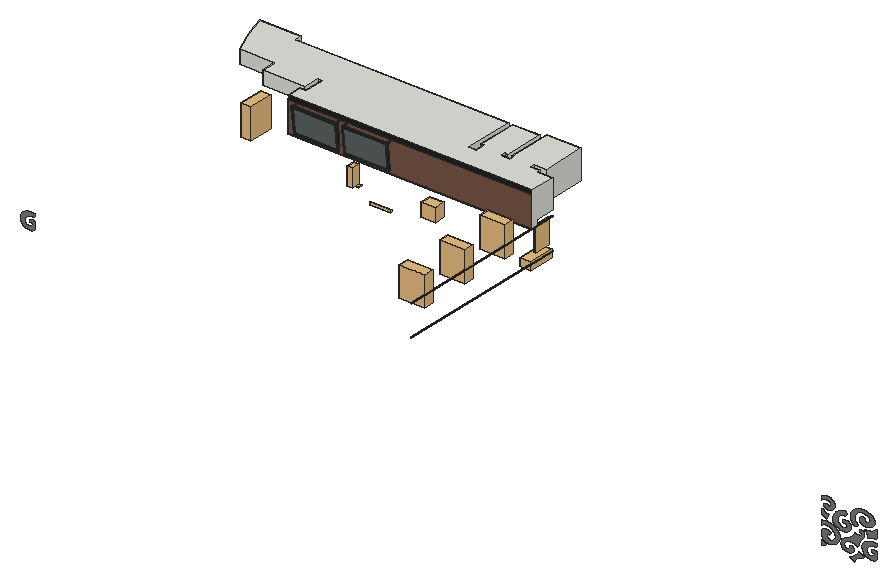
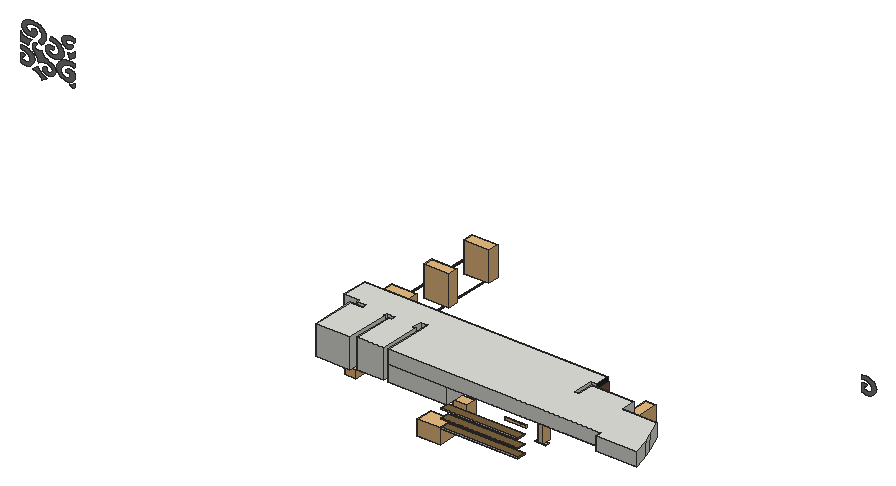
# SketchUp Ruby script. Lengths in inches.
U = 1.inch
M = Sketchup.active_model
def pt(a) = Geom::Point3d.new(a.map { |v| v * U })
def face(e, loops, mat)
  f = e.add_face(loops[0].map { |a| pt(a) })
  loops[1..].each { |l| e.add_face(l.map { |a| pt(a) }).erase! }
  f.material = f.back_material = mat if mat
  f
end
# faces: each face lists its corners as indices into pts; further lists are holes
def faces(e, pts, list, mat = nil) = list.each { |f| face(e, (f[0].is_a?(Array) ? f : [f]).map { |l| l.map { |i| pts[i] } }, mat) }
# xy, xz, yz: faces in a plane at the given z, y or x. An outline is a flat list of corners, or four numbers for a rectangle; further outlines are holes
def ring(l) = l.size == 4 ? [[l[0], l[1]], [l[2], l[1]], [l[2], l[3]], [l[0], l[3]]] : l.each_slice(2).to_a
def flat(e, list, mat, &to3) = list.each { |f| face(e, (f[0].is_a?(Array) ? f : [f]).map { |l| ring(l).map { |u, v| to3.(u, v) } }, mat) }
def xy(e, z, list, mat = nil) = flat(e, list, mat) { |x, y| [x, y, z] }
def xz(e, y, list, mat = nil) = flat(e, list, mat) { |x, z| [x, y, z] }
def yz(e, x, list, mat = nil) = flat(e, list, mat) { |y, z| [x, y, z] }
def lines(e, pts, list) = list.each { |a, b| e.add_line(pt(pts[a]), pt(pts[b])) }
# prism: a flat outline (further loops are holes) pulled along v
def prism(e, loops, v, mat = nil)
  f = face(e, loops, mat); d = Geom::Vector3d.new(v.map { |x| x * U })
  f.pushpull(f.normal.samedirection?(d) ? d.length : -d.length)
end
def box(e, o, s, mat = nil) = prism(e, [[o, [o[0] + s[0], o[1], o[2]], [o[0] + s[0], o[1] + s[1], o[2]], [o[0], o[1] + s[1], o[2]]]], [0, 0, s[2]], mat)
def at(x, y, z, deg = 0) = Geom::Transformation.translation(pt([x, y, z])) * Geom::Transformation.rotation(ORIGIN, Z_AXIS, deg.degrees)
def axes(o, x, y, z) = Geom::Transformation.new([*x, 0, *y, 0, *z, 0, *pt(o).to_a, 1])
def part(name) = M.definitions.add(name)
# library, detail: a bought-in or finely detailed component or shape, given as its bounding box
def library(name, o, s) = part(name).tap { |d| box(d.entities, o, s) }
def detail(e, o, s) = box(e.add_group.entities, o, s)
def put(e, d, t, mat = nil) = e.add_instance(d, t).tap { |i| i.material = mat if mat }
def group(e, t, mat = nil) = e.add_group.tap { |g| g.transformation = t; g.material = mat if mat }.entities
root = M.entities
M.materials.add("Floor board").color = [119, 86, 70]
M.materials.add("Floor board2").color = [119, 86, 70]
M.materials.add("Image2").color = [96, 104, 104]
M.materials.add("Material31 copy1").color = [126, 98, 61]
M.materials.add("Small-Wooden-Floor").color = [116, 79, 55]
M.materials.add("Sophie_Shoes2").color = [35, 35, 35]
M.materials.add("[0043_SaddleBrown]4").color = [124, 123, 122]
M.materials.add("[Metal_Corrogated_Shiny]2").color = [193, 193, 193]
c1 = library("Group\#90",[0,0,0],[37.3,15.24,44.88])
c2 = part("Group\#62")
box(c2.entities,[0,-3.9375,0],[1.97,3.9375,1.97],"Sophie_Shoes2")
c3 = part("Component\#73")
detail(c3.entities,[0,0,-0.5],[5.95,16.95,0.625])
c4 = part("omponent_2\#3")
xy(c4.entities,0.125,[[[0.47,0.47,5.47,16.47],[1.375,15.02,4.5625,15.45],[1.375,14.15,4.5625,14.59],[1.375,13.29,4.5625,13.72],[1.375,12.43,4.5625,12.86],[1.375,11.5625,4.5625,12],[1.375,10.7,4.5625,11.13],[1.375,9.84,4.5625,10.27],[1.375,8.97,4.5625,9.41],[1.375,8.11,4.5625,8.54],[1.375,7.25,4.5625,7.68],[1.375,6.38,4.5625,6.82],[1.375,5.52,4.5625,5.95],[1.375,4.66,4.5625,5.09],[1.375,3.79,4.5625,4.23],[1.375,2.93,4.5625,3.36],[1.375,2.07,4.5625,2.5],[1.375,1.26,4.5625,1.64]]],"[Metal_Corrogated_Shiny]2")
put(c4.entities,c3,at(0,0,0))
c5 = library("Cobra Beer Dispense Font",[-3.83,-2.55,-1.15],[8.17,12.19,26.9])
c6 = part("Group\#60")
xy(c6.entities,0,[[-106.3,12.99,7.875,25.59]])
xy(c6.entities,1.97,[[-106.3,12.99,7.875,25.59]],"Material31 copy1")
xz(c6.entities,12.99,[[-106.3,0,7.875,1.97]],"Material31 copy1")
xz(c6.entities,25.59,[[-106.3,0,7.875,1.97]])
yz(c6.entities,-106.3,[[12.99,0,25.59,1.97]],"Material31 copy1")
yz(c6.entities,7.875,[[12.99,0,25.59,1.97]],"Material31 copy1")
c7 = library("IKEA FINTORP-",[6.23,0.25,8.28],[1.42,31.37,3.33])
c8 = library("maq caf expresso 2 mdulos",[-0.08,-0.31,0.08],[34.26,25.22,21.95])
c9 = library("ZJ8P4AC",[-1.97,-16.1,36],[20.97,16.1,19.66])
c10 = library("Group\#93",[0,0,0],[37.3,15.24,44.88])
c11 = library("Group\#94",[0,0,0],[37.3,15.24,44.88])
c12 = library("Group\#105",[0,0,0],[37.34,15.24,44.88])
c13 = library("Group\#84",[0,-1.97,0],[16.33,39.37,11.37])
c14 = library("Group\#83",[-2.91,0,0],[33.89,3.125,48.37])
xz(root,589.17,[[4168.05,173.83,4167.56,174.24,4167.0625,174.64,4166.54,175.02,4166,175.39,4165.4375,175.74,4164.86,176.08,4164.26,176.4,4163.65,176.71,4163.02,177,4162.38,177.27,4161.73,177.53,4161.0625,177.77,4162.625,178.34,4164.13,178.99,4165.5625,179.72,4166.92,180.52,4168.2,181.39,4169.39,182.32,4170.48,183.31,4171.47,184.35,4172.36,185.44,4173.14,186.58,4173.8,187.75,4174.35,188.95,4174.9,188.49,4175.46,188.03,4176.03,187.59,4176.61,187.15,4177.2,186.72,4177.8,186.29,4178.42,185.87,4179.04,185.46,4179.66,185.06,4180.3,184.66,4180.95,184.27,4181.61,183.89,4179.94,183.57,4178.33,183.14,4176.79,182.59,4175.33,181.94,4173.96,181.19,4172.71,180.35,4171.57,179.42,4170.57,178.41,4169.71,177.34,4168.99,176.21,4168.44,175.04],[4119.85,179.89,4119.85,185.26,4120.27,184.92,4120.7,184.6,4121.16,184.3,4121.63,184.01,4122.125,183.73,4122.63,183.47,4123.15,183.23,4123.69,183,4124.24,182.79,4124.81,182.6,4125.38,182.42,4125.97,182.27,4125.59,181.9375,4125.17,181.63,4124.73,181.34,4124.27,181.07,4123.77,180.83,4123.26,180.61,4122.72,180.42,4122.17,180.26,4121.61,180.12,4121.03,180.02,4120.44,179.9375],[4157.27,183.24,4155.84,183.36,4154.45,183.65,4153.14,184.08,4151.93,184.65,4150.86,185.34,4149.94,186.15,4149.21,187.04,4148.67,188.01,4148.34,189.02,4148.23,190.0625,4148.12,191.26,4148.18,192.46,4148.42,193.65,4148.82,194.8125,4149.39,195.9375,4150.11,197.02,4150.99,198.04,4152.01,198.99,4153.16,199.85,4154.43,200.63,4155.81,201.31,4157.27,201.88,4158.66,202.4,4159.99,202.99,4161.27,203.65,4162.47,204.37,4163.6,205.15,4164.65,205.98,4165.62,206.87,4166.5,207.81,4167.28,208.78,4167.96,209.8,4168.55,210.85,4169.02,211.92,4169.7,211.55,4170.44,211.25,4171.23,211.03,4172.06,210.88,4172.9,210.82,4173.75,210.84,4174.59,210.9375,4175.4,211.12,4176.17,211.38,4176.88,211.72,4177.53,212.12,4178.09,212.58,4178.3,212.95,4178.44,213.33,4178.53,213.73,4178.55,214.13,4178.51,214.53,4178.41,214.92,4178.25,215.3,4178.03,215.67,4177.75,216.02,4177.42,216.34,4177.04,216.63,4176.62,216.89,4176.39,217.04,4176.21,217.23,4176.08,217.43,4176,217.65,4175.99,217.875,4176.04,218.1,4176.15,218.3125,4176.32,218.5,4176.53,218.67,4176.78,218.8,4177.07,218.9,4177.37,218.95,4177.93,218.98,4178.48,218.95,4179.03,218.86,4179.55,218.72,4180.04,218.52,4180.48,218.28,4180.875,217.99,4181.21,217.67,4181.47,217.3125,4181.66,216.9375,4181.78,216.54,4181.82,216.14,4182.03,215.47,4182.18,214.79,4182.25,214.11,4182.26,213.42,4182.2,212.73,4182.07,212.05,4181.87,211.38,4181.6,210.72,4181.27,210.08,4180.87,209.45,4180.41,208.85,4179.89,208.27,4178.96,207.26,4178.09,206.23,4177.28,205.16,4176.54,204.07,4175.88,202.95,4175.28,201.82,4174.76,200.67,4174.3,199.5,4173.93,198.32,4173.625,197.12,4173.4,195.92,4173.25,194.71,4172.28,195.61,4171.16,196.41,4169.9,197.09,4168.54,197.66,4167.08,198.09,4165.56,198.375,4163.99,198.52,4162.42,198.52,4160.86,198.37,4159.34,198.07,4157.88,197.63,4156.52,197.0625,4155.54,196.53,4154.68,195.9,4153.93,195.2,4153.31,194.44,4152.83,193.625,4152.5,192.77,4152.32,191.9,4152.31,191.01,4152.45,190.14,4152.75,189.28,4153.19,188.46,4153.78,187.68,4154.33,187.38,4154.93,187.15,4155.57,186.98,4156.24,186.89,4156.93,186.87,4157.61,186.92,4158.27,187.04,4158.89,187.24,4159.48,187.5,4160,187.82,4160.44,188.1875,4160.8125,188.6,4160.69,188.9,4160.6,189.2,4160.55,189.5,4160.53,189.81,4160.55,190.12,4160.59,190.42,4160.67,190.72,4160.79,191.02,4160.94,191.31,4161.11,191.59,4161.32,191.86,4161.56,192.11,4161.79,192.31,4162.0625,192.48,4162.37,192.61,4162.7,192.71,4163.05,192.77,4163.4,192.79,4163.76,192.77,4164.11,192.71,4164.44,192.61,4164.75,192.48,4165.02,192.31,4165.25,192.11,4165.92,191.31,4166.4,190.43,4166.65,189.51,4166.6875,188.57,4166.5,187.63,4166.09,186.74,4165.48,185.91,4164.68,185.17,4163.71,184.53,4162.61,184.03,4161.41,183.66,4160.14,183.45,4158.72,183.27],[4130,184.38,4128.84,184.54,4127.71,184.78,4126.61,185.09,4125.5625,185.48,4124.57,185.94,4123.64,186.47,4122.78,187.05,4122.01,187.69,4121.32,188.38,4120.73,189.12,4120.24,189.89,4119.85,190.7,4119.85,198.78,4120.38,199.6875,4121.16,200.5,4122.14,201.17,4123.3,201.69,4124.58,202.03,4125.93,202.17,4127.29,202.12,4128.61,201.86,4129.82,201.42,4130.89,200.8,4131.76,200.05,4132.4,199.18,4132.49,198.97,4132.54,198.75,4132.55,198.53,4132.51,198.32,4132.42,198.1,4132.3,197.9,4132.13,197.72,4131.93,197.55,4131.7,197.41,4131.44,197.3,4131.16,197.21,4130.87,197.15,4130.14,197.24,4129.4,197.23,4128.68,197.13,4128,196.93,4127.38,196.64,4126.84,196.28,4126.41,195.85,4126.09,195.37,4125.9,194.85,4125.85,194.32,4125.93,193.8,4126.15,193.29,4126.33,192.63,4126.65,192,4127.11,191.41,4127.69,190.88,4128.38,190.43,4129.16,190.06,4130.01,189.78,4130.91,189.6,4131.84,189.53,4132.77,189.5625,4133.68,189.7,4134.55,189.9375,4135.91,190.72,4137.1,191.64,4138.09,192.67,4138.88,193.79,4139.4375,194.98,4139.75,196.21,4139.83,197.47,4139.65,198.72,4139.24,199.93,4138.58,201.1,4137.71,202.18,4136.63,203.17,4136.19,203.82,4135.68,204.45,4135.1,205.04,4134.45,205.59,4133.74,206.1,4132.97,206.57,4132.15,206.99,4131.29,207.37,4130.39,207.68,4129.45,207.94,4128.48,208.15,4127.5,208.3,4126.8,208.36,4126.09,208.375,4125.39,208.35,4124.6875,208.28,4124,208.17,4123.32,208.02,4122.67,207.83,4122.04,207.6,4121.4375,207.33,4120.87,207.03,4120.34,206.69,4119.85,206.32,4119.85,211.9,4122,212.41,4124.21,212.74,4126.47,212.875,4128.73,212.8125,4130.96,212.56,4133.14,212.11,4135.22,211.48,4137.1875,210.67,4139.01,209.7,4140.65,208.58,4142.1,207.33,4143.32,205.96,4144.99,203.92,4146.15,201.7,4146.76,199.375,4146.81,197.01,4146.28,194.67,4145.21,192.43,4143.62,190.36,4141.5625,188.51,4139.09,186.95,4136.28,185.72,4133.22,184.86],[2942.18,185,2940.82,185.0625,2939.48,185.24,2938.1875,185.54,2936.95,185.94,2935.8,186.46,2934.74,187.07,2933.84,187.69,2933.01,188.36,2932.24,189.0625,2931.53,189.8,2930.9,190.57,2930.34,191.375,2929.86,192.2,2929.45,193.05,2929.125,193.92,2928.88,194.79,2928.72,195.68,2928.64,196.58,2928.75,198.46,2929.26,200.32,2930.15,202.09,2931.4,203.75,2932.98,205.26,2934.86,206.58,2936.99,207.67,2939.33,208.53,2941.82,209.12,2944.4,209.4375,2947.02,209.47,2949.62,209.22,2949.62,204.51,2947.39,204.57,2945.18,204.34,2943.06,203.84,2941.09,203.08,2939.33,202.09,2937.84,200.89,2936.66,199.53,2935.83,198.03,2935.37,196.46,2935.3,194.85,2935.62,193.26,2936.3125,191.73,2937.11,191.08,2938.06,190.54,2939.13,190.15,2940.29,189.91,2941.49,189.83,2942.7,189.91,2943.85,190.16,2944.93,190.55,2945.875,191.09,2946.67,191.75,2947.28,192.5,2947.68,193.32,2947.75,193.65,2947.74,193.99,2947.66,194.32,2947.49,194.64,2947.25,194.93,2946.95,195.19,2946.59,195.4,2946.1875,195.57,2945.75,195.6875,2945.29,195.75,2944.82,195.75,2944.36,195.7,2944.12,195.77,2943.89,195.87,2943.68,195.98,2943.48,196.11,2943.31,196.25,2943.15,196.41,2943.03,196.58,2942.92,196.75,2942.85,196.93,2942.8,197.12,2942.78,197.3125,2942.79,197.5,2943.15,197.89,2943.59,198.24,2944.09,198.54,2944.64,198.8,2945.23,199,2945.85,199.14,2946.49,199.22,2947.14,199.24,2947.79,199.19,2948.43,199.09,2949.04,198.93,2949.62,198.7,2949.62,187.07,2948.55,186.46,2947.4,185.94,2946.16,185.54,2944.87,185.24,2943.53,185.0625],
  [4192.8,185,4191.44,185.0625,4190.11,185.24,4188.8125,185.54,4187.58,185.94,4186.42,186.46,4185.36,187.07,4184.47,187.69,4183.63,188.36,4182.86,189.0625,4182.16,189.8,4181.53,190.57,4180.97,191.375,4180.48,192.2,4180.08,193.05,4179.75,193.92,4179.51,194.79,4179.34,195.68,4179.26,196.58,4179.38,198.46,4179.89,200.32,4180.78,202.09,4182.03,203.75,4183.61,205.26,4185.49,206.58,4187.62,207.67,4189.95,208.53,4192.44,209.12,4195.03,209.4375,4197.64,209.47,4200.24,209.22,4200.24,204.51,4198.01,204.57,4195.8,204.34,4193.68,203.84,4191.71,203.08,4189.96,202.09,4188.47,200.89,4187.29,199.53,4186.46,198.03,4186,196.46,4185.92,194.85,4186.24,193.26,4186.9375,191.73,4187.73,191.08,4188.68,190.54,4189.76,190.15,4190.92,189.91,4192.12,189.83,4193.32,189.91,4194.48,190.16,4195.55,190.55,4196.5,191.09,4197.29,191.75,4197.9,192.5,4198.3,193.32,4198.375,193.65,4198.37,193.99,4198.28,194.32,4198.12,194.64,4197.88,194.93,4197.58,195.19,4197.22,195.4,4196.8125,195.57,4196.375,195.6875,4195.91,195.75,4195.45,195.75,4194.98,195.7,4194.74,195.77,4194.51,195.87,4194.3,195.98,4194.11,196.11,4193.93,196.25,4193.78,196.41,4193.65,196.58,4193.55,196.75,4193.47,196.93,4193.42,197.12,4193.4,197.3125,4193.41,197.5,4193.78,197.89,4194.22,198.24,4194.71,198.54,4195.26,198.8,4195.85,199,4196.48,199.14,4197.12,199.22,4197.77,199.24,4198.42,199.19,4199.05,199.09,4199.67,198.93,4200.24,198.7,4200.24,187.07,4199.18,186.46,4198.02,185.94,4196.79,185.54,4195.49,185.24,4194.16,185.0625],[4150.69,208.61,4148.36,208.71,4146.07,209.07,4143.89,209.68,4141.87,210.53,4140.0625,211.6,4138.5,212.86,4137.24,214.28,4136.29,215.82,4135.69,217.45,4135.45,219.125,4135.58,220.81,4136.07,222.46,4136.625,224.06,4137.38,225.62,4138.33,227.12,4139.47,228.55,4140.79,229.9,4142.27,231.16,4143.91,232.31,4145.69,233.35,4147.59,234.27,4149.6,235.06,4151.7,235.71,4153.875,236.22,4154.29,235.77,4154.65,235.31,4154.96,234.82,4155.23,234.32,4155.4375,233.81,4155.59,233.28,4155.69,232.75,4155.74,232.22,4155.73,231.68,4155.66,231.15,4155.54,230.62,4155.37,230.1,4154.01,230.21,4152.65,230.19,4151.31,230.04,4150.01,229.75,4148.78,229.33,4147.63,228.8,4146.61,228.16,4145.71,227.42,4144.96,226.6,4144.38,225.71,4143.97,224.77,4143.75,223.8,4143.38,222.89,4143.15,221.95,4143.0625,221,4143.12,220.05,4143.31,219.11,4143.64,218.19,4144.11,217.3,4144.7,216.45,4145.42,215.65,4146.26,214.91,4147.19,214.24,4148.23,213.65,4149.18,213.25,4150.23,212.99,4151.32,212.875,4152.43,212.91,4153.5,213.1,4154.51,213.43,4155.41,213.89,4156.18,214.46,4156.78,215.13,4157.19,215.875,4157.41,216.66,4157.41,217.45,4157.32,217.85,4157.16,218.23,4156.93,218.59,4156.63,218.92,4156.28,219.23,4155.86,219.49,4155.41,219.71,4154.91,219.89,4154.39,220.01,4153.85,220.09,4153.29,220.1,4152.74,220.07,4152.17,220.05,4151.61,220.13,4151.08,220.3,4150.62,220.55,4150.25,220.86,4150,221.23,4149.86,221.63,4149.86,222.05,4149.98,222.45,4150.23,222.83,4150.59,223.15,4151.04,223.4,4152.29,223.84,4153.63,224.12,4155.01,224.21,4156.39,224.12,4157.73,223.85,4158.98,223.4,4160.09,222.81,4161.04,222.07,4161.78,221.23,4162.31,220.3,4162.58,219.32,4162.61,218.32,4162.66,217.11,4162.49,215.9,4162.08,214.72,4161.46,213.6,4160.625,212.54,4159.6,211.58,4158.4,210.73,4157.05,210.01,4155.58,209.42,4154.01,208.99,4152.37,208.72],[4188.26,213.07,4188.16,213.85,4188,214.62,4187.78,215.39,4187.52,216.14,4187.2,216.89,4186.82,217.625,4186.4,218.34,4185.93,219.05,4185.4,219.73,4184.83,220.4,4184.22,221.04,4183.56,221.66,4185.21,221.55,4186.87,221.5625,4188.52,221.7,4190.14,221.96,4191.72,222.33,4193.24,222.82,4194.68,223.41,4196.03,224.11,4197.27,224.91,4198.39,225.79,4199.39,226.75,4200.24,227.78,4200.24,215.23,4199.2,215.21,4198.17,215.16,4197.13,215.08,4196.1,214.98,4195.08,214.84,4194.07,214.67,4193.07,214.47,4192.08,214.25,4191.1,213.99,4190.14,213.71,4189.1875,213.41],[4127.19,216.375,4126.5,216.63,4125.81,216.91,4125.14,217.2,4124.48,217.52,4123.84,217.84,4123.22,218.1875,4122.61,218.54,4122.02,218.92,4121.45,219.31,4120.89,219.71,4120.36,220.125,4119.85,220.56,4119.85,227.67,4120.37,227.04,4120.96,226.43,4121.62,225.86,4122.34,225.34,4123.11,224.85,4123.94,224.42,4124.82,224.03,4125.73,223.7,4126.68,223.42,4127.66,223.2,4128.66,223.04,4129.68,222.93,4129.26,222.44,4128.875,221.9375,4128.53,221.42,4128.22,220.89,4127.95,220.35,4127.72,219.79,4127.53,219.23,4127.38,218.67,4127.27,218.1,4127.21,217.52,4127.18,216.95],[4167.64,220.74,4166.52,221.82,4165.51,222.95,4164.62,224.13,4163.85,225.36,4163.22,226.63,4162.71,227.92,4162.35,229.24,4162.11,230.58,4162.02,231.92,4162.07,233.27,4162.25,234.61,4162.57,235.94,4163.1,237.37,4163.83,238.75,4164.75,240.07,4165.86,241.32,4167.13,242.48,4168.57,243.55,4170.14,244.5,4171.84,245.33,4173.65,246.03,4175.55,246.59,4177.52,247.02,4179.54,247.29,4181.74,247.4,4183.94,247.29,4186.1,246.97,4188.18,246.4375,4190.14,245.71,4191.95,244.79,4193.56,243.71,4194.96,242.47,4196.11,241.12,4196.99,239.66,4197.59,238.125,4197.89,236.55,4197.89,235.18,4197.61,233.83,4197.05,232.52,4196.24,231.29,4195.18,230.15,4193.91,229.14,4192.44,228.27,4190.82,227.57,4189.07,227.04,4187.23,226.71,4185.34,226.57,4183.45,226.63,4181.97,226.85,4180.57,227.24,4179.27,227.79,4178.12,228.48,4177.14,229.3,4176.36,230.23,4175.79,231.23,4175.47,232.29,4175.39,233.37,4175.55,234.45,4175.96,235.49,4176.6,236.47,4177.12,236.87,4177.73,237.18,4178.42,237.39,4179.16,237.5,4179.91,237.49,4180.65,237.375,4181.34,237.15,4181.94,236.83,4182.45,236.43,4182.82,235.96,4183.06,235.44,4182.95,235.09,4182.89,234.73,4182.88,234.37,4182.9375,234.01,4183.05,233.65,4183.21,233.3125,4183.43,232.98,4183.69,232.68,4184,232.39,4184.36,232.13,4184.75,231.91,4185.17,231.71,4186.18,231.82,4187.16,232.03,4188.08,232.35,4188.92,232.77,4189.66,233.28,4190.29,233.86,4190.78,234.5,4191.13,235.19,4191.33,235.91,4191.375,236.65,4191.26,237.38,4190.99,238.09,4190.25,239.28,4189.24,240.36,4187.99,241.3,4186.54,242.08,4184.9375,242.67,4183.22,243.07,4181.43,243.25,4179.62,243.21,4177.85,242.96,4176.16,242.5,4174.6,241.84,4173.22,241,4171.77,239.82,4170.55,238.51,4169.57,237.1,4168.87,235.6,4168.4375,234.06,4168.29,232.48,4168.4375,230.91,4168.87,229.36,4169.57,227.86,4170.55,226.45,4171.77,225.14,4173.22,223.96,4172.86,223.61,4172.47,223.28,4172.07,222.95,4171.64,222.65,4171.2,222.35,4170.74,222.07,4170.26,221.81,4169.76,221.5625,4169.25,221.33,4168.73,221.12,4168.19,220.92],
  [4129.7,229.18,4128.42,229.23,4127.17,229.45,4126.01,229.84,4124.97,230.38,4124.08,231.06,4123.39,231.84,4122.92,232.7,4122.68,233.61,4122.59,233.96,4122.59,234.32,4122.7,234.67,4122.89,235,4123.17,235.29,4123.52,235.54,4123.93,235.74,4124.39,235.875,4124.88,235.94,4125.375,235.94,4125.86,235.87,4126.32,235.73,4126.59,235.48,4126.875,235.24,4127.18,235.01,4127.51,234.8,4127.86,234.6,4128.22,234.42,4128.6,234.26,4128.99,234.11,4129.39,233.98,4129.81,233.87,4130.23,233.78,4130.66,233.71,4131.22,234.05,4131.72,234.45,4132.15,234.89,4132.5,235.36,4132.77,235.86,4132.95,236.375,4133.04,236.91,4133.05,237.44,4132.96,237.97,4132.78,238.49,4132.51,238.99,4132.16,239.46,4131.4375,240.18,4130.55,240.79,4129.54,241.29,4128.42,241.65,4127.23,241.875,4126.01,241.95,4124.78,241.875,4123.6,241.65,4122.48,241.29,4121.46,240.79,4120.58,240.18,4119.85,239.46,4119.85,244.71,4120.73,245.16,4121.66,245.55,4122.64,245.87,4123.66,246.125,4124.7,246.3,4125.77,246.41,4126.85,246.4375,4127.92,246.39,4128.99,246.27,4130.03,246.08,4131.04,245.8125,4132.01,245.48,4133.71,244.68,4135.21,243.71,4136.47,242.57,4137.46,241.3,4138.15,239.93,4138.54,238.5,4138.6,237.04,4138.33,235.6,4137.75,234.2,4136.87,232.89,4135.71,231.7,4134.29,230.65,4133.3125,230.05,4132.2,229.6,4130.98,229.3]],"[0043_SaddleBrown]4")
p = [[3451.42,661.35,234.52],[3451.42,661.35,235.3],[4183.14,589.17,234.9],[4183.06,589.17,235.44],[4119.85,589.17,176.23],[4119.85,589.17,179.89]]
lines(root,p,[[0,1],[2,3],[4,5]])
put(root,c1,at(3047.58,868.72,217.78,90))
g1 = group(root,at(3099.24,879.1,238.5625))
put(g1,c2,at(0,5.9,37.38))
g2 = group(g1,at(0,5.94,0.2))
yz(g2,0,[[-1.96,-0.2,-5.94,38.95,-3.98,39.15,0,0]],"Sophie_Shoes2")
yz(g2,1.97,[[-2.16,1.76,-1.96,1.78,-5.54,37.01,-5.74,36.99]],"Sophie_Shoes2")
yz(g2,64.96,[[-2.16,1.76,-5.74,36.99,-5.54,37.01,-1.96,1.78]],"Sophie_Shoes2")
yz(g2,66.93,[[-1.96,-0.2,0,0,-3.98,39.15,-5.94,38.95]],"Sophie_Shoes2")
p = [[0,-1.96,-0.2],[66.93,-1.96,-0.2],[66.93,-5.94,38.95],[0,-5.94,38.95],[64.96,-5.74,36.99],[64.96,-2.16,1.76],
  [1.97,-2.16,1.76],[1.97,-5.74,36.99],[0,0,0],[66.93,0,0],[0,-3.98,39.15],[66.93,-3.98,39.15],
  [64.96,-1.96,1.78],[64.96,-5.54,37.01],[1.97,-5.54,37.01],[1.97,-1.96,1.78]]
faces(g2,p,[[[0,1,2,3],[4,5,6,7]],[8,9,1,0],[9,8,10,11],[6,5,12,15],[4,7,14,13],[11,10,3,2]],"Sophie_Shoes2")
faces(g2,p,[[12,13,14,15]],"Image2")
put(g1,c2,at(64.96,5.9,37.38))
put(root,c4,at(3159.91,913.9375,184.3125,-90))
put(root,c5,at(3168.59,903.45,185.47))
put(root,c6,at(3244.25,967.04,208.73))
put(root,c6,at(3244.25,967.04,221.13))
put(root,c6,at(3244.25,967.04,234.32))
g3 = group(root,at(3173.89,879.1,238.5625))
put(g3,c2,at(0,5.9,37.38))
g4 = group(g3,at(0,5.94,0.2))
yz(g4,0,[[-1.96,-0.2,-5.94,38.95,-3.98,39.15,0,0]],"Sophie_Shoes2")
yz(g4,1.97,[[-2.16,1.76,-1.96,1.78,-5.54,37.01,-5.74,36.99]],"Sophie_Shoes2")
yz(g4,64.96,[[-2.16,1.76,-5.74,36.99,-5.54,37.01,-1.96,1.78]],"Sophie_Shoes2")
yz(g4,66.93,[[-1.96,-0.2,0,0,-3.98,39.15,-5.94,38.95]],"Sophie_Shoes2")
p = [[0,-1.96,-0.2],[66.93,-1.96,-0.2],[66.93,-5.94,38.95],[0,-5.94,38.95],[64.96,-5.74,36.99],[64.96,-2.16,1.76],
  [1.97,-2.16,1.76],[1.97,-5.74,36.99],[0,0,0],[66.93,0,0],[0,-3.98,39.15],[66.93,-3.98,39.15],
  [64.96,-1.96,1.78],[64.96,-5.54,37.01],[1.97,-5.54,37.01],[1.97,-1.96,1.78]]
faces(g4,p,[[[0,1,2,3],[4,5,6,7]],[8,9,1,0],[9,8,10,11],[6,5,12,15],[4,7,14,13],[11,10,3,2]],"Sophie_Shoes2")
faces(g4,p,[[12,13,14,15]],"Image2")
put(g3,c2,at(64.96,5.9,37.38))
g5 = group(root,at(3099.26,906.02,286.68))
xy(g5,-52.36,[[[-9.84,-21.65,-9.84,0,0,0,0,-11.8125,352.95,-11.8125,352.95,-21.65],[0,-20.47,195.18,-12.99]]],"Sophie_Shoes2")
xy(g5,-51.38,[[-9.84,-21.65,-9.25,0],[-9.25,-21.65,352.95,-21.0625]],"Sophie_Shoes2")
xy(g5,-51.18,[[-9.84,-21.65,-9.84,0,-9.25,0,-9.25,-21.0625,352.95,-21.0625,352.95,-21.65]],"Floor board")
xy(g5,-51.18,[[0,-12.4,145.18,-11.8125]],"Sophie_Shoes2")
xy(g5,-50.59,[[0,-12.4,145.18,-11.8125]])
xy(g5,-47.64,[[0,-20.47,195.18,-12.99]],"Sophie_Shoes2")
xy(g5,-43.31,[[145.18,-11.8125,145.18,86.61,231.79,86.61,231.79,13.78,242,13.78,242,27.56,237.7,27.56,237.7,86.61,277.8,86.61,277.8,27.56,273.49,27.56,273.49,21.65,285.85,21.65,285.85,27.56,283.7,27.56,283.7,92.52,335.25,92.52,335.25,27.56,317.35,27.56,317.35,21.65,330.23,21.65,330.23,17.19,352.95,17.19,352.95,-11.8125]])
xy(g5,-19.69,[[0,-11.8125,0,29.53,-5.91,29.53,-5.91,5.91,-68.9,5.91,-68.9,27.62,-120.71,27.62,-132.65,55.86,-137.96,70.69,-145.4,96.46,-84.48,96.46,-84.48,86.61,145.18,86.61,145.18,-11.8125]])
xy(g5,-6.3,[[-9.84,-21.65,352.95,-20.87],[-9.84,-20.87,-9.06,0]],"Small-Wooden-Floor")
xy(g5,0,[[-9.06,-20.87,352.95,-20.87,352.95,17.19,330.23,17.19,330.23,21.65,317.35,21.65,317.35,27.56,335.25,27.56,335.25,92.52,283.7,92.52,283.7,27.56,285.85,27.56,285.85,21.65,273.49,21.65,273.49,27.56,277.8,27.56,277.8,86.61,237.7,86.61,237.7,27.56,242,27.56,242,13.78,231.79,13.78,231.79,86.61,-84.48,86.61,-84.48,96.46,-145.4,96.46,-137.96,70.69,-132.65,55.86,-120.71,27.62,-68.9,27.62,-68.9,5.91,-5.91,5.91,-5.91,29.53,0,29.53,0,0,-9.06,0]])
xz(g5,-21.65,[[-9.84,-51.18,352.95,-6.3]],"Floor board")
xz(g5,-21.65,[[-9.84,-52.36,352.95,-51.38]],"Sophie_Shoes2")
xz(g5,-21.0625,[[-9.25,-51.38,352.95,-51.18]],"Sophie_Shoes2")
xz(g5,-20.87,[[-9.06,-6.3,352.95,0]],"Sophie_Shoes2")
xz(g5,-20.47,[[0,-52.36,195.18,-47.64]])
xz(g5,-12.99,[[0,-52.36,195.18,-47.64]],"Sophie_Shoes2")
xz(g5,-12.4,[[0,-51.18,145.18,-50.59]],"Sophie_Shoes2")
xz(g5,-11.8125,[[0,-50.59,145.18,-19.69]])
xz(g5,-11.8125,[[0,-52.36,0,-51.18,145.18,-51.18,145.18,-43.31,352.95,-43.31,352.95,-52.36]],"Sophie_Shoes2")
xz(g5,0,[[-9.84,-52.36,-9.84,-51.38,-9.25,-51.38,-9.25,-51.18,-9.84,-51.18,-9.84,-6.3,-9.06,-6.3,-9.06,0,0,0,0,-52.36]])
xz(g5,5.91,[[-68.9,-19.69,-5.91,0]])
xz(g5,13.78,[[231.79,-43.31,242,0]])
xz(g5,17.19,[[330.23,-43.31,352.95,0]])
xz(g5,21.65,[[273.49,-43.31,285.85,0],[317.35,-43.31,330.23,0]])
xz(g5,27.56,[[237.7,-43.31,242,0],[273.49,-43.31,277.8,0],[283.7,-43.31,285.85,0],[317.35,-43.31,335.25,0]])
xz(g5,27.62,[[-120.71,-19.69,-68.9,0]])
xz(g5,29.53,[[-5.91,-19.69,0,0]])
xz(g5,86.61,[[145.18,-43.31,231.79,-19.69],[237.7,-43.31,277.8,0],[-84.48,-19.69,231.79,0]])
xz(g5,92.52,[[283.7,-43.31,335.25,0]])
xz(g5,96.46,[[-145.4,-19.69,-84.48,0]])
yz(g5,-84.48,[[86.61,-19.69,96.46,0]])
yz(g5,-68.9,[[5.91,-19.69,27.62,0]])
yz(g5,-9.84,[[-21.65,-51.18,0,-6.3]],"Floor board2")
yz(g5,-9.84,[[-21.65,-52.36,0,-51.38]],"Sophie_Shoes2")
yz(g5,-9.25,[[-21.0625,-51.38,0,-51.18]],"Sophie_Shoes2")
yz(g5,-9.06,[[-20.87,-6.3,0,0]],"Sophie_Shoes2")
yz(g5,-5.91,[[5.91,-19.69,29.53,0]])
yz(g5,0,[[-11.8125,-52.36,0,-52.36,0,-19.69,-11.8125,-19.69,-11.8125,-50.59,-12.4,-50.59,-12.4,-51.18,-11.8125,-51.18],[0,-19.69,29.53,0]])
yz(g5,0,[[-20.47,-52.36,-12.99,-47.64]],"Sophie_Shoes2")
yz(g5,145.18,[[-12.4,-51.18,-11.8125,-50.59],[-11.8125,-43.31,86.61,-19.69]])
yz(g5,195.18,[[-20.47,-52.36,-12.99,-47.64]],"Sophie_Shoes2")
yz(g5,231.79,[[13.78,-43.31,86.61,-19.69],[13.78,-19.69,86.61,0]])
yz(g5,237.7,[[27.56,-43.31,86.61,0]])
yz(g5,242,[[13.78,-43.31,27.56,0]])
yz(g5,273.49,[[21.65,-43.31,27.56,0]])
yz(g5,277.8,[[27.56,-43.31,86.61,0]])
yz(g5,283.7,[[27.56,-43.31,92.52,0]])
yz(g5,285.85,[[21.65,-43.31,27.56,0]])
yz(g5,317.35,[[21.65,-43.31,27.56,0]])
yz(g5,330.23,[[17.19,-43.31,21.65,0]])
yz(g5,335.25,[[27.56,-43.31,92.52,0]])
yz(g5,352.95,[[-21.65,-52.36,-11.8125,-52.36,-11.8125,-43.31,17.19,-43.31,17.19,0,-20.87,0,-20.87,-6.3,-21.65,-6.3,-21.65,-51.18,-21.0625,-51.18,-21.0625,-51.38,-21.65,-51.38]])
p = [[-120.71,27.62,0],[-132.65,55.86,0],[-132.65,55.86,-19.69],[-120.71,27.62,-19.69],[-137.96,70.69,0],[-137.96,70.69,-19.69],
  [-145.4,96.46,0],[-145.4,96.46,-19.69],[352.95,-21.65,-6.3],[362.91,-21.65,-6.3]]
faces(g5,p,[[0,1,2,3],[1,4,5,2],[4,6,7,5]])
lines(g5,p,[[8,9]])
put(root,c7,at(3239.64,883.01,172,90))
put(root,c8,at(3254.18,967.04,186.29))
put(root,c9,at(3292,903.22,144.38,180))
put(root,c10,at(3414.27,760.66,217.12))
put(root,c11,at(3414.27,835.46,217.12))
put(root,c12,at(3414.27,685.85,217.12))
put(root,c13,at(3435.09,885.81,180.38))
put(root,c14,axes([3452.1,893.69,200.98],[0,0.73,0],[-0.73,0,0],[0,0,0.73]))
g6 = group(root,at(3451.42,700.19,188.26))
prism(g6,[[[0,-38.84,0.2],[0,-38.84,0],[0.79,-38.84,0],[0.79,-38.84,1.18],[0,-38.84,1.18],[0,-38.84,0.98],[0.59,-38.84,0.98],[0.59,-38.84,0.2]]],[0,261.86,0],"Sophie_Shoes2")
g7 = group(root,at(3451.42,661.35,234.32))
prism(g7,[[[0,0,0.2],[0,0,0],[0.79,0,0],[0.79,0,1.18],[0,0,1.18],[0,0,0.98],[0.59,0,0.98],[0.59,0,0.2]]],[0,261.86,0],"Sophie_Shoes2")
